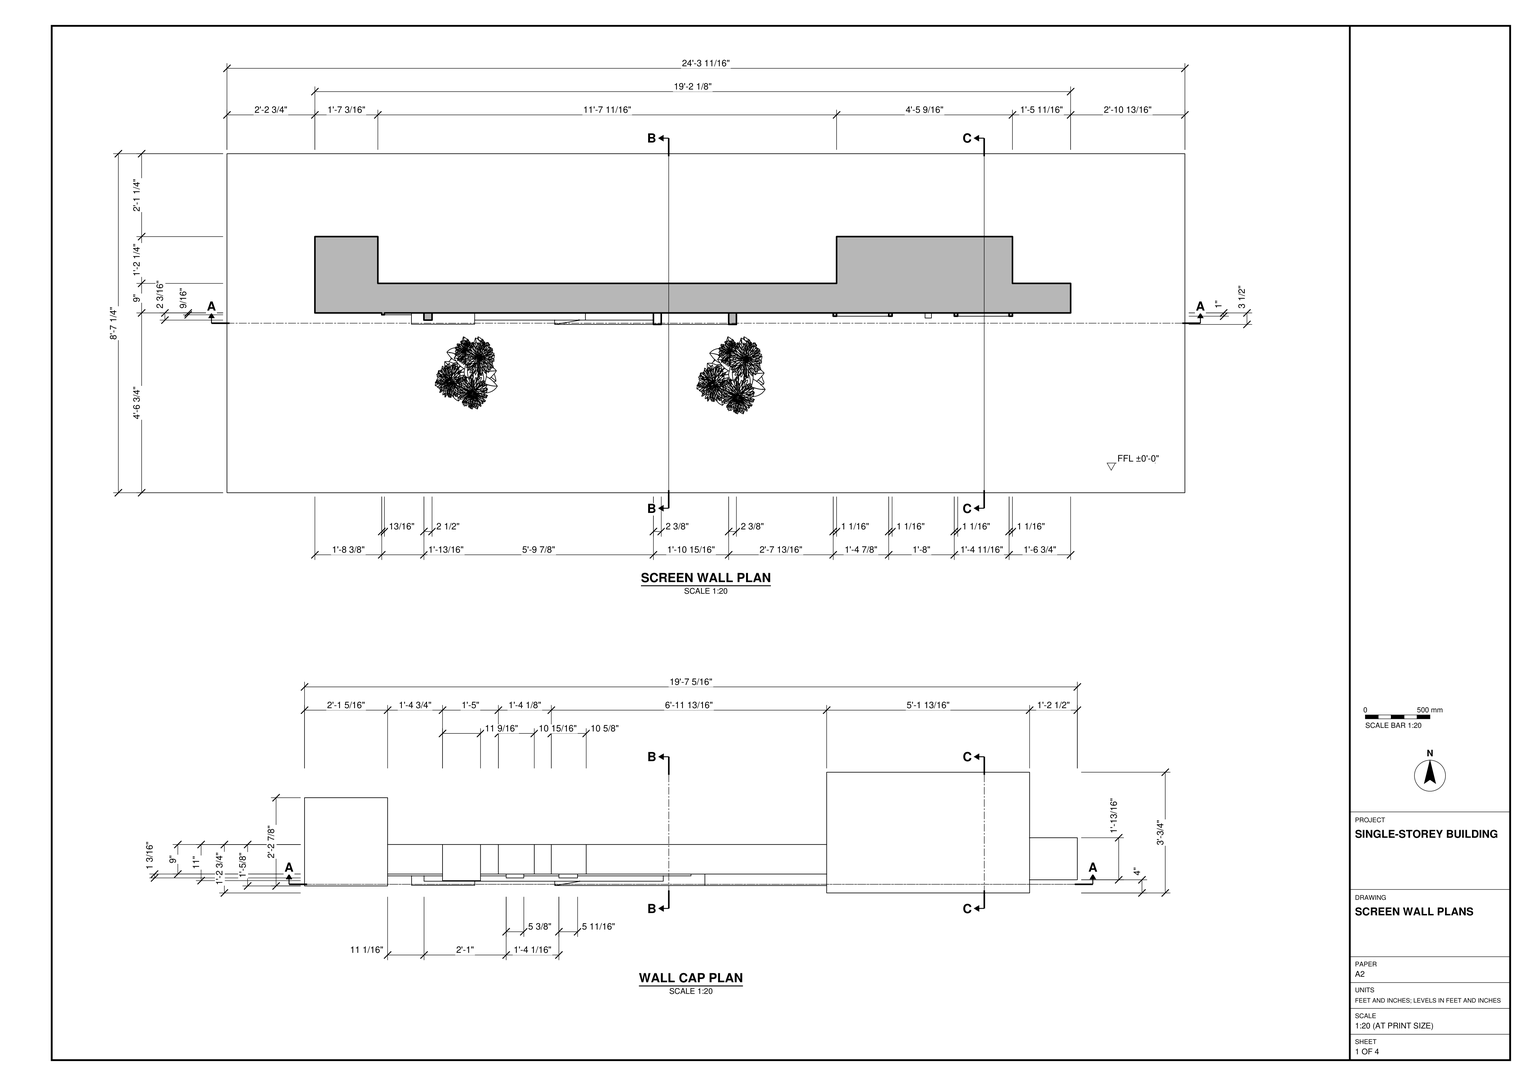
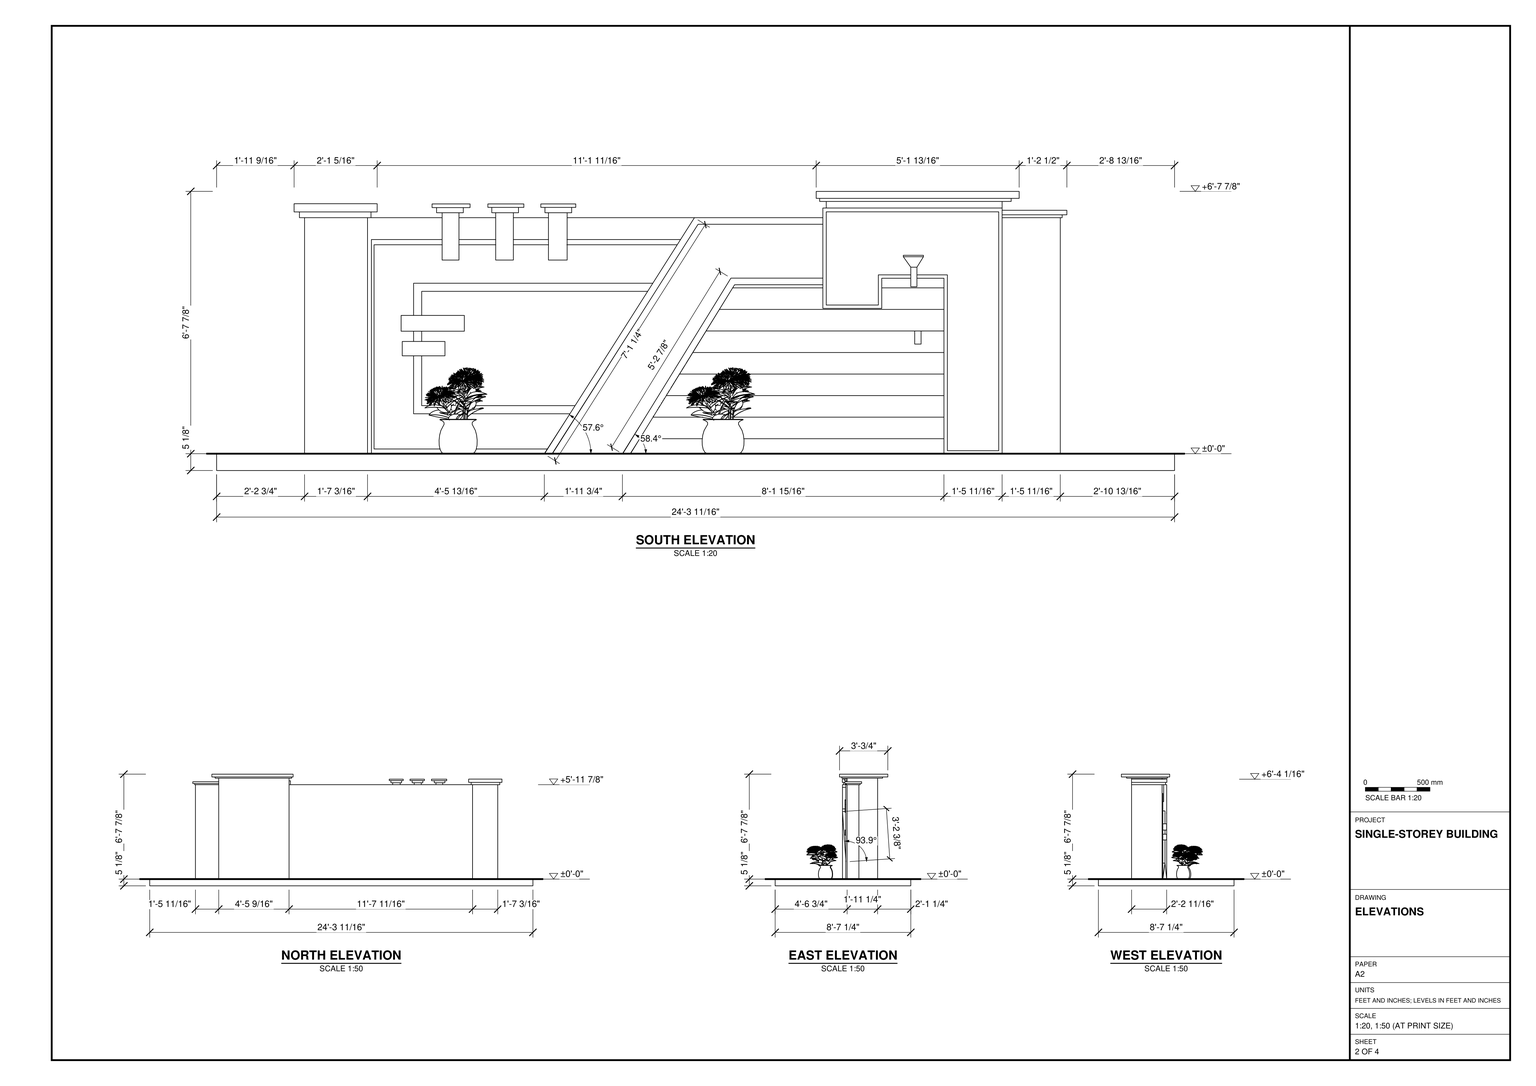
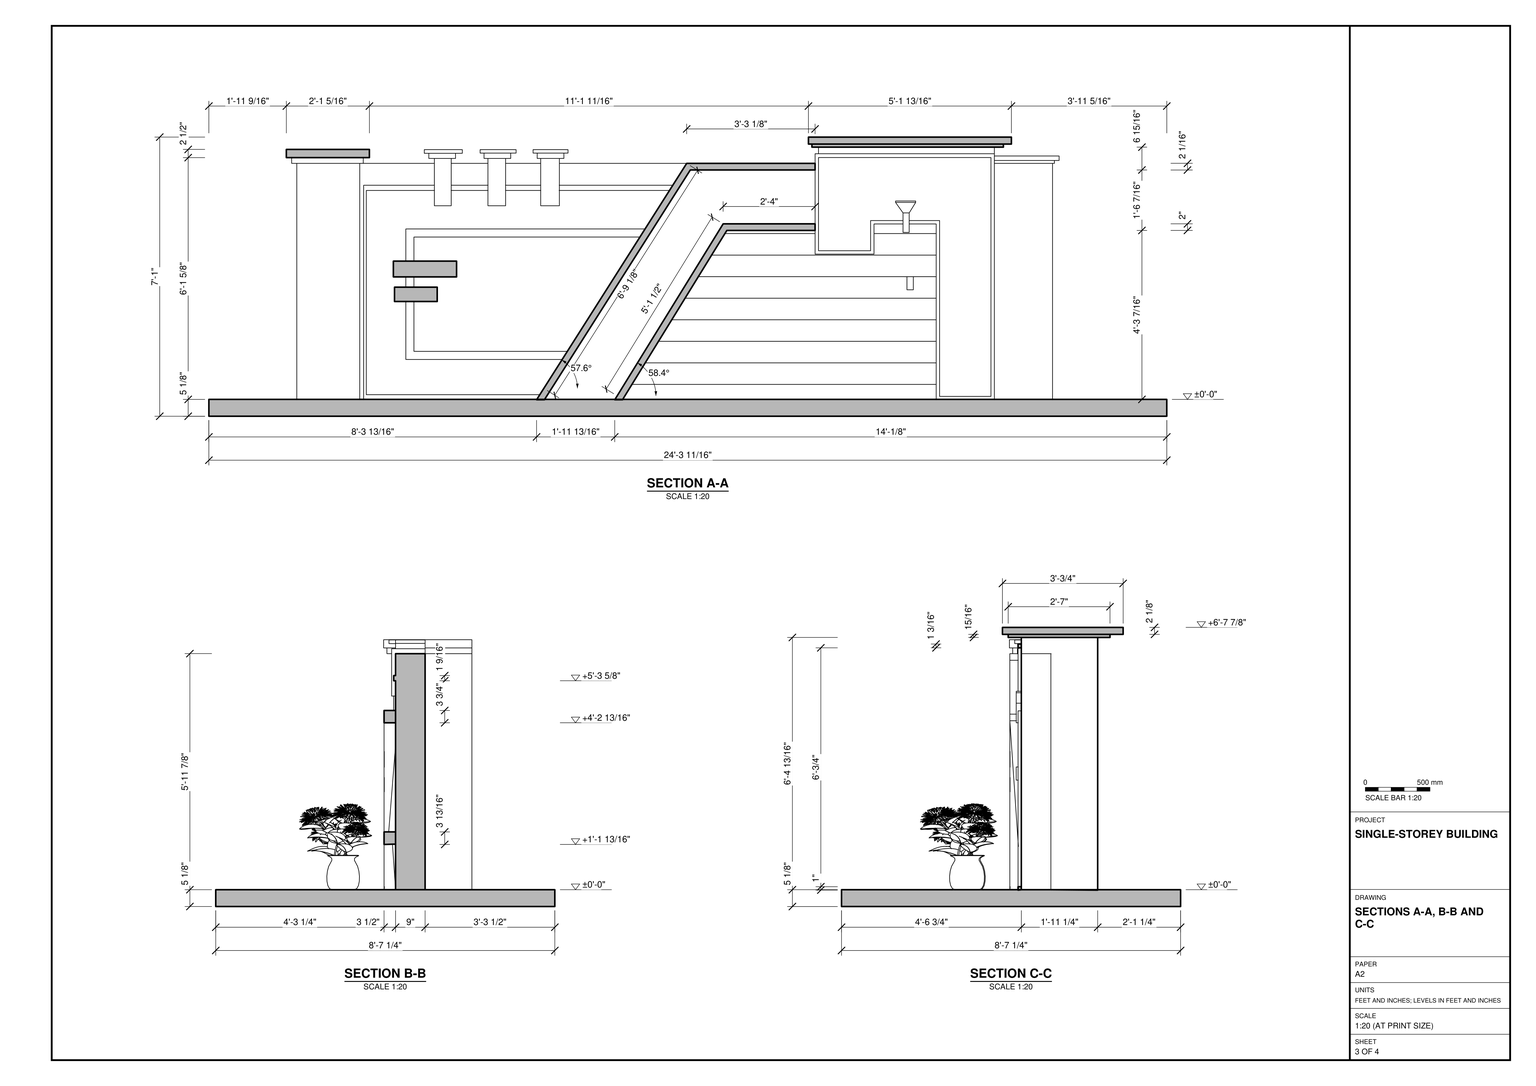
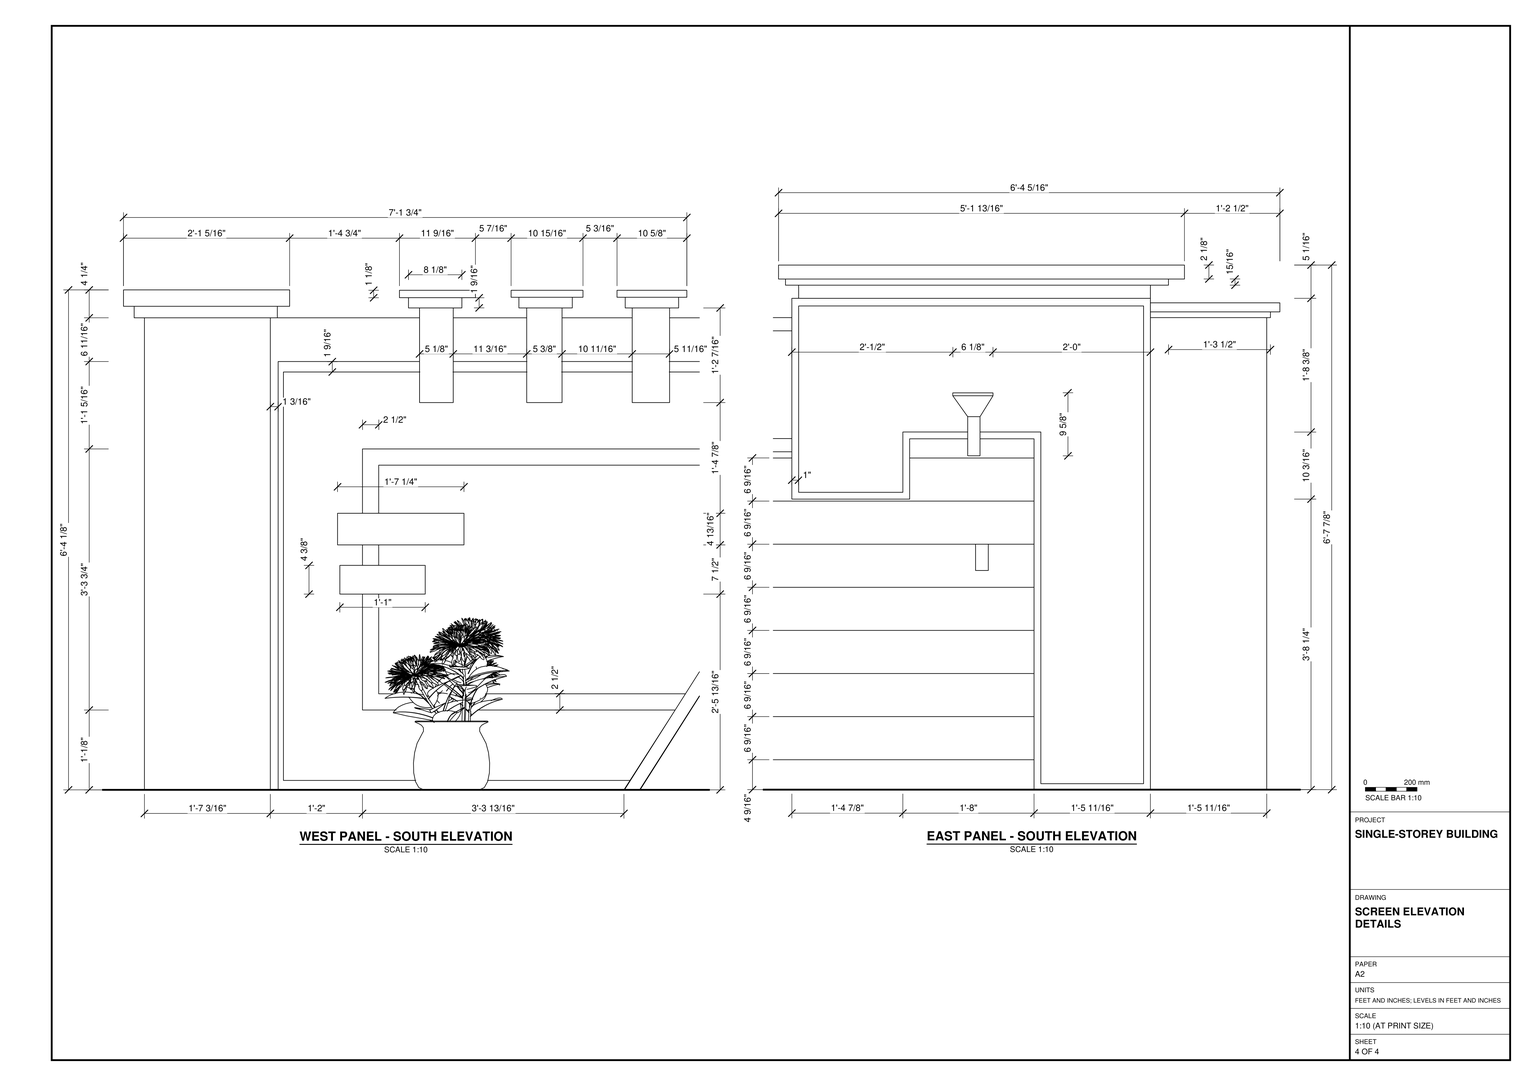
Build the screen wall and its base in SketchUp using task_files/diagram_01.pdf. Work in feet and inches. Set the top of the slab at the finished ground level of ±0'-0". The overall model is 24'-3 11/16" long, 8'-7 1/4" deep and 7'-1" high, measured from the underside of the slab to the top of the highest wall cap.

Use the screen wall plan to locate the wall on the slab and set its thicknesses. The narrow wall is deeper at the left pier and at the broad pier near the right end. Use the separate cap plan and the sections to model the cap overhangs and changes in height. On the south face, form the outlined left panel, its two short projecting bars and the three capped vertical strips above it. Run the broad diagonal band up from the slab and turn it horizontally toward the broad pier. Fit the horizontal courses beneath it to the diagonal edge and the stepped outline of the pier.

Place the two potted plants on the slab in front of the wall as shown in plan. Decor and loose items such as the plants may be any suitable library components. Keep the slab, wall and applied details in separate groups or components, and use components for repeated parts. Save one SketchUp model as output_files/freestanding_screen_wall_on_a_rectangular_slab.skp.

# SketchUp Ruby script. Lengths in inches.
U = 1.inch
M = Sketchup.active_model
def pt(a) = Geom::Point3d.new(a.map { |v| v * U })
def face(e, loops, mat)
  f = e.add_face(loops[0].map { |a| pt(a) })
  loops[1..].each { |l| e.add_face(l.map { |a| pt(a) }).erase! }
  f.material = f.back_material = mat if mat
  f
end
# faces: each face lists its corners as indices into pts; further lists are holes
def faces(e, pts, list, mat = nil) = list.each { |f| face(e, (f[0].is_a?(Array) ? f : [f]).map { |l| l.map { |i| pts[i] } }, mat) }
# xy, xz, yz: faces in a plane at the given z, y or x. An outline is a flat list of corners, or four numbers for a rectangle; further outlines are holes
def ring(l) = l.size == 4 ? [[l[0], l[1]], [l[2], l[1]], [l[2], l[3]], [l[0], l[3]]] : l.each_slice(2).to_a
def flat(e, list, mat, &to3) = list.each { |f| face(e, (f[0].is_a?(Array) ? f : [f]).map { |l| ring(l).map { |u, v| to3.(u, v) } }, mat) }
def xy(e, z, list, mat = nil) = flat(e, list, mat) { |x, y| [x, y, z] }
def xz(e, y, list, mat = nil) = flat(e, list, mat) { |x, z| [x, y, z] }
def yz(e, x, list, mat = nil) = flat(e, list, mat) { |y, z| [x, y, z] }
def lines(e, pts, list) = list.each { |a, b| e.add_line(pt(pts[a]), pt(pts[b])) }
# prism: a flat outline (further loops are holes) pulled along v
def prism(e, loops, v, mat = nil)
  f = face(e, loops, mat); d = Geom::Vector3d.new(v.map { |x| x * U })
  f.pushpull(f.normal.samedirection?(d) ? d.length : -d.length)
end
def box(e, o, s, mat = nil) = prism(e, [[o, [o[0] + s[0], o[1], o[2]], [o[0] + s[0], o[1] + s[1], o[2]], [o[0], o[1] + s[1], o[2]]]], [0, 0, s[2]], mat)
def at(x, y, z, deg = 0) = Geom::Transformation.translation(pt([x, y, z])) * Geom::Transformation.rotation(ORIGIN, Z_AXIS, deg.degrees)
def axes(o, x, y, z) = Geom::Transformation.new([*x, 0, *y, 0, *z, 0, *pt(o).to_a, 1])
def part(name) = M.definitions.add(name)
# library, detail: a bought-in or finely detailed component or shape, given as its bounding box
def library(name, o, s) = part(name).tap { |d| box(d.entities, o, s) }
def detail(e, o, s) = box(e.add_group.entities, o, s)
def put(e, d, t, mat = nil) = e.add_instance(d, t).tap { |i| i.material = mat if mat }
def group(e, t, mat = nil) = e.add_group.tap { |g| g.transformation = t; g.material = mat if mat }.entities
root = M.entities
M.materials.add("[Carrera Marble]").color = [207, 207, 207]
M.materials.add("[Color C08]").color = [102, 51, 0]
M.materials.add("[Concrete Aggregate Smoke]").color = [154, 150, 148]
c1 = library("VASO COM FLORES",[0.59,-0.39,0],[11.65,11.91,19.45])
xy(root,3.0625,[[0,0,291.6875,103.25]],"[Concrete Aggregate Smoke]")
xy(root,8.1875,[[99.78,54.1875,102.16,54.75,99.78,54.75]])
xy(root,8.1875,[[[0,0,291.6875,103.25],[47.13,54.1875,47.13,54.75,26.77,54.75,26.77,78,45.94,78,45.94,63.75,256.9,63.75,256.9,54.75,102.16,54.75,99.78,54.1875]],[47.13,54.1875,99.78,54.1875,99.78,54.75,256.9,54.75,256.9,63.75,45.94,63.75,45.94,78,26.77,78,26.77,54.75,47.13,54.75]],"[Concrete Aggregate Smoke]")
xy(root,9.1,[[222.51,53.75,238.15,54.75]])
xy(root,9.62,[[47.9375,54.1875,100.77,54.75]])
xy(root,20.34,[[59.97,52.5625,107.58,54.75]])
xy(root,22.8125,[[62.44,52.5625,109.14,54.75]])
xy(root,37.99,[[56.53,51.3125,56.53,54.75,59.97,54.75,59.97,52.5625,62.44,52.5625,62.44,54.75,69.53,54.75,69.53,51.3125]])
xy(root,41.5625,[[212.57,53.1875,214.51,54.75]],"[Carrera Marble]")
xy(root,42.37,[[56.53,51.3125,69.53,51.3125,69.53,54.75,62.44,54.75,62.44,52.5625,59.97,52.5625,59.97,54.75,56.53,54.75]])
xy(root,45.48,[[56.18,51.3125,56.18,54.75,59.97,54.75,59.97,52.5625,62.44,52.5625,62.44,54.75,75.43,54.75,75.43,51.3125]])
xy(root,45.5625,[[212.57,53.1875,214.51,54.75]],"[Carrera Marble]")
xy(root,50.3,[[56.18,51.3125,75.43,51.3125,75.43,54.75,62.44,54.75,62.44,52.5625,59.97,52.5625,59.97,54.75,56.18,54.75]])
xy(root,52.43,[[184.6,53.75,202.53,54.75]])
xy(root,53.46,[[185.63,53.75,201.5,54.75]])
xy(root,57.625,[[62.44,52.5625,131.24,54.75]])
xy(root,59.02,[[211.37,53.1875,213.25,54.75]],"[Carrera Marble]")
xy(root,59.64,[[157.72,51.25,184.6,54.75]])
xy(root,60.09,[[59.97,52.5625,132.8125,54.75]])
xy(root,61.61,[[202.53,53.75,211.37,54.75],[211.37,53.75,213.25,54.75],[213.25,53.75,221.47,54.75]])
xy(root,61.65,[[156.6,51.25,184.6,54.75]])
xy(root,62.65,[[201.5,53.75,211.37,54.75],[211.37,53.75,213.25,54.75],[213.25,53.75,222.51,54.75]])
xy(root,64.98,[[211.37,53.1875,213.25,54.75]])
xy(root,67.15,[[68.66,53.5625,73.79,54.625],[84.98,53.5625,90.36,54.75],[101.04,53.5625,106.73,54.75]])
xy(root,68.17,[[209.1,53.1875,215.22,54.75]])
xy(root,68.61,[[209.1,53.1875,215.22,54.75]],"[Carrera Marble]")
xy(root,71.8125,[[47.9375,54.1875,47.9375,54.75,140.25,54.75,140.25,54.1875,73.79,54.1875,73.79,54.625,68.66,54.625,68.66,54.1875],[68.66,54.1875,73.79,54.625]])
xy(root,73.4,[[47.13,54.1875,68.66,54.75],[68.66,54.1875,73.79,54.75],[73.79,54.1875,141.26,54.75]])
xy(root,78.05,[[146.6,51.25,184.6,54.75]])
xy(root,80.0625,[[145.49,51.25,184.6,54.75],[25.21,54.75,26.77,78],[26.77,54.75,26.77,78,45.94,78,45.94,63.75,47.01,63.75,47.01,54.75],[47.01,54.75,68.66,63.75],[68.66,54.75,73.79,63.75],
  [73.79,54.75,84.98,63.75],[84.98,54.75,90.36,63.75],[90.36,54.75,101.04,63.75],[101.04,54.75,106.73,63.75],[106.73,54.75,185.63,63.75],
  [45.94,63.75,47.01,78]])
xy(root,80.0625,[[25.21,52.125,45.94,54.75],[45.94,52.125,47.01,54.75],[239.18,54.1875,257.46,54.75],[239.18,54.75,256.9,63.75],[256.9,54.75,257.46,64.6875],
  [239.18,63.75,256.9,64.6875]],"[Carrera Marble]")
xy(root,80.9375,[[239.18,53,239.18,54.1875,257.46,54.1875,257.46,64.6875,239.18,64.6875,239.18,65.8125,258.9,65.8125,258.9,53],[239.18,54.1875,257.46,64.6875]],"[Carrera Marble]")
xy(root,81.5625,[[68.66,53.5625,73.79,54.75],[84.98,53.5625,90.36,54.75],[101.04,53.5625,106.73,54.75],[68.66,54.75,73.79,63.75],[84.98,54.75,90.36,63.75],
  [101.04,54.75,106.73,63.75]])
xy(root,81.5625,[[66.98,54.75,68.66,63.75],[73.79,54.75,75.11,63.75],[83.79,54.75,84.98,63.75],[90.36,54.75,91.92,63.75],[99.98,54.75,101.04,63.75],
  [106.73,54.75,108.11,63.75]],"[Carrera Marble]")
xy(root,81.8125,[[25.21,52.125,47.01,78]])
xy(root,81.8125,[[23.59,51.125,23.59,78,25.21,78,25.21,52.125,26.77,52.125,26.77,51.125],[26.77,51.125,45.94,52.125],[45.94,51.125,45.94,52.125,47.01,52.125,47.01,78,48.88,78,48.88,51.125]],"[Carrera Marble]")
xy(root,81.84,[[185.63,53.75,238.15,54.75]])
xy(root,82.3125,[[239.18,53,258.9,65.8125]],"[Carrera Marble]")
xy(root,83,[[184.6,53.75,239.18,54.75]])
xy(root,83.125,[[66.98,54.75,75.11,63.75]])
xy(root,83.125,[[65.6,52.75,77.17,54.75],[65.6,54.75,66.98,63.75],[75.11,54.75,77.17,63.75]],"[Carrera Marble]")
xy(root,83.1875,[[83.79,54.75,91.92,63.75],[99.98,54.75,108.11,63.75]])
xy(root,83.1875,[[82.6,54.75,83.79,63.75],[91.92,54.75,93.54,63.75],[98.73,54.75,99.98,63.75],[108.11,54.75,109.36,63.75]],"[Carrera Marble]")
xy(root,84.25,[[65.6,52.75,77.17,63.75],[82.6,54.75,93.54,63.75],[98.73,54.75,109.36,63.75]],"[Carrera Marble]")
xy(root,84.3125,[[23.59,51.125,48.88,78]],"[Carrera Marble]")
xy(root,85,[[185.63,54.75,239.18,78]])
xy(root,85,[[[183.63,50.75,241.93,81.75],[185.63,54.75,239.18,78]]],"[Carrera Marble]")
xy(root,85.9375,[[183.63,50.75,241.93,81.75]])
xy(root,85.9375,[[[182.57,49,244.37,85.75],[183.63,50.75,241.93,81.75]]],"[Carrera Marble]")
xy(root,88.0625,[[182.57,49,244.37,85.75]],"[Carrera Marble]")
xz(root,0,[[0,3.0625,291.6875,8.1875]],"[Concrete Aggregate Smoke]")
xz(root,49,[[182.57,85.9375,244.37,88.0625]],"[Carrera Marble]")
xz(root,50.75,[[183.63,85,241.93,85.9375]],"[Carrera Marble]")
xz(root,51.125,[[23.59,81.8125,48.88,84.3125]],"[Carrera Marble]")
xz(root,51.25,[[99.78,8.0625,102.16,8.0625,146.6,78.05,184.6,78.05,184.6,80.0625,145.49,80.0625],[123.58,8.0625,125.95,8.0625,157.72,59.64,184.6,59.64,184.6,61.65,156.6,61.65]])
xz(root,51.3125,[[56.53,37.99,69.53,42.37],[56.18,45.48,75.43,50.3]])
xz(root,52.125,[[25.21,80.0625,47.01,81.8125]],"[Carrera Marble]")
xz(root,52.5625,[[59.97,20.34,107.58,20.34,109.14,22.8125,62.44,22.8125,62.44,37.99,59.97,37.99],[59.97,37.99,62.44,42.37],[59.97,42.37,62.44,45.48],[59.97,45.48,62.44,50.3],[59.97,50.3,62.44,50.3,62.44,57.625,131.24,57.625,131.92,58.6875,132.8125,60.09,59.97,60.09]])
xz(root,52.75,[[65.6,83.125,77.17,84.25]],"[Carrera Marble]")
xz(root,53,[[239.18,80.9375,258.9,82.3125]],"[Carrera Marble]")
xz(root,53.1875,[[212.57,41.5625,214.51,45.5625],[211.37,59.02,213.25,64.98],[211.37,64.98,213.25,64.98,215.22,68.17,209.1,68.17],[209.1,68.17,215.22,68.61]],"[Carrera Marble]")
xz(root,53.5625,[[68.66,67.15,73.79,81.5625],[84.98,67.15,90.36,81.5625],[101.04,67.15,106.73,81.5625]],"[Carrera Marble]")
xz(root,53.75,[[221.47,8.0625,239.18,8.0625,239.18,83,184.6,83,184.6,52.43,202.53,52.43,202.53,61.61,211.37,61.61,211.37,62.65,201.5,62.65,201.5,53.46,185.63,53.46,185.63,81.84,238.15,81.84,238.15,9.1,222.51,9.1,222.51,62.65,213.25,62.65,213.25,61.61,221.47,61.61],[211.37,61.61,213.25,62.65]])
xz(root,54.1875,[[47.13,8.1875,99.78,8.1875,100.77,9.62,47.9375,9.62,47.9375,71.8125,68.66,71.8125,68.66,73.4,47.13,73.4],[68.66,71.8125,73.79,73.4],[73.79,71.8125,140.25,71.8125,141.26,73.4,73.79,73.4]])
xz(root,54.1875,[[239.18,80.0625,257.46,80.9375]],"[Carrera Marble]")
xz(root,54.625,[[68.66,67.15,73.79,71.8125]])
xz(root,54.75,[[45.94,8.1875,47.13,8.1875,47.13,73.4,68.66,73.4,68.66,80.0625,45.94,80.0625],[99.78,8.1875,100.77,9.62,107.58,20.34,109.14,22.8125,131.24,57.625,131.92,58.6875,134.3,58.6875,130.13,52.125,102.16,8.1875],[123.58,8.1875,130.51,19.3125,132.82,19.3125,125.95,8.1875],[125.95,8.1875,132.82,19.3125,132.875,19.3125,128.83,12.75],[125.95,8.1875,221.47,8.1875,221.47,12.75,128.83,12.75],
  [221.47,8.1875,221.47,61.61,202.53,61.61,202.53,58.6875,201.5,58.6875,201.5,62.65,222.51,62.65,222.51,9.1,238.15,9.1,238.15,81.84,186.61,81.84,186.61,83,239.18,83,239.18,8.1875],[128.83,12.75,221.47,12.75,221.47,19.3125,132.875,19.3125],[130.51,19.3125,134.56,25.875,136.87,25.875,132.82,19.3125],[132.82,19.3125,136.87,25.875,136.92,25.875,132.875,19.3125],[132.875,19.3125,221.47,19.3125,221.47,25.875,136.92,25.875],
  [59.97,20.34,59.97,37.99,62.44,37.99,62.44,22.8125,109.14,22.8125,107.58,20.34],[134.56,25.875,138.6,32.4375,140.92,32.4375,136.87,25.875],[136.87,25.875,140.92,32.4375,140.96,32.4375,136.92,25.875],[136.92,25.875,221.47,25.875,221.47,32.4375,140.96,32.4375],[138.6,32.4375,142.64,39,144.97,39,140.92,32.4375],
  [140.92,32.4375,144.97,39,145.01,39,140.96,32.4375],[140.96,32.4375,221.47,32.4375,221.47,39,145.01,39],[56.53,37.99,59.97,42.37],[59.97,37.99,62.44,42.37],[62.44,37.99,69.53,42.37],
  [142.64,39,146.6875,45.5625,149.03,45.5625,144.97,39],[144.97,39,149.03,45.5625,149.05,45.5625,145.01,39],[145.01,39,221.47,39,221.47,45.5625,214.51,45.5625,214.51,41.5625,212.57,41.5625,212.57,45.5625,149.05,45.5625],[212.57,41.5625,214.51,45.5625],[59.97,42.37,62.44,46.3],
  [56.18,45.48,59.97,50.3],[62.44,45.48,75.43,50.3],[146.6875,45.5625,150.73,52.125,153.08,52.125,149.03,45.5625],[149.03,45.5625,153.08,52.125,153.09,52.125,149.05,45.5625],[149.05,45.5625,221.47,45.5625,221.47,52.125,153.09,52.125],
  [59.97,46.3,62.44,50.3],[59.97,50.3,59.97,60.09,132.8125,60.09,131.92,58.6875,131.24,57.625,62.44,57.625,62.44,50.3],[150.73,52.125,154.77,58.6875,157.13,58.6875,153.08,52.125],[153.08,52.125,157.13,58.6875,157.14,58.6875,153.09,52.125],[153.08,52.125,157.13,58.6875,157.72,59.64,157.14,58.6875,153.09,52.125],
  [153.09,52.125,221.47,52.125,221.47,58.6875,202.53,58.6875,202.53,52.43,184.6,52.43,184.6,58.6875,157.14,58.6875],[184.6,52.43,184.6,58.6875,185.63,58.6875,185.63,53.46,201.5,53.46,201.5,58.6875,202.53,58.6875,202.53,52.43],[131.92,58.6875,132.8125,60.09,136.08,65.25,138.47,65.25,134.3,58.6875],[154.77,58.6875,156.6,61.65,184.6,61.65,184.6,59.64,157.72,59.64,157.13,58.6875],[157.13,58.6875,157.72,59.64,157.14,58.6875],
  [157.14,58.6875,184.6,58.6875,184.6,59.64,157.72,59.64],[184.6,58.6875,185.63,59.64],[202.53,58.6875,221.47,58.6875,221.47,61.61,213.25,61.61,213.25,59.02,211.37,59.02,211.37,61.61,202.53,61.61],[184.6,59.64,185.63,65.25],[211.37,62.65,213.25,64.98],
  [211.37,64.98,209.1,68.17,215.22,68.17,213.25,64.98],[136.08,65.25,140.25,71.8125,142.63,71.8125,138.47,65.25],[184.6,65.25,185.63,71.8125],[84.98,67.15,90.36,71.8125],[101.04,67.15,106.73,71.8125],
  [209.1,68.17,215.22,68.61],[84.98,71.8125,90.36,73.4],[101.04,71.8125,106.73,73.4],[140.25,71.8125,141.26,73.4,145.49,80.0625,184.6,80.0625,184.6,78.05,146.6,78.05,142.63,71.8125],[184.6,71.8125,185.63,80.0625],
  [68.66,73.4,73.79,80.0625],[73.79,73.4,84.98,80.0625],[84.98,73.4,90.36,80.0625],[90.36,73.4,101.04,80.0625],[101.04,73.4,106.73,80.0625],
  [106.73,73.4,141.26,73.4,145.49,80.0625,106.73,80.0625],[184.6,80.0625,185.63,83],[185.63,81.84,186.61,83]])
xz(root,54.75,[[26.77,8.1875,45.94,80.0625],[239.18,8.1875,256.9,80.0625],[62.44,22.8125,109.14,22.8125,131.24,57.625,62.44,57.625,62.44,50.3,75.43,50.3,75.43,45.48,62.44,45.48,62.44,42.37,69.53,42.37,69.53,37.99,62.44,37.99],[66.98,81.5625,75.11,83.125],[83.79,81.5625,91.92,83.1875],
  [99.98,81.5625,108.11,83.1875],[185.63,83,239.18,85],[82.6,83.1875,93.54,84.25],[98.73,83.1875,109.36,84.25]],"[Carrera Marble]")
xz(root,54.75,[[102.16,8.1875,123.58,8.1875,130.51,19.3125,134.56,25.875,142.64,39,146.6875,45.5625,150.73,52.125,154.77,58.6875,156.6,61.65,184.6,61.65,184.6,78.05,146.6,78.05,142.63,71.8125,138.47,65.25,130.13,52.125],[222.51,9.1,238.15,9.1,238.15,81.84,185.63,81.84,185.63,53.46,201.5,53.46,201.5,62.65,211.37,62.65,211.37,64.98,209.1,68.17,209.1,68.61,215.22,68.61,215.22,68.17,213.25,64.98,213.25,62.65,222.51,62.65],[47.9375,9.62,100.77,9.62,107.58,20.34,59.97,20.34,59.97,37.99,56.53,37.99,56.53,42.37,59.97,42.37,59.97,45.48,56.18,45.48,56.18,50.3,59.97,50.3,59.97,60.09,132.8125,60.09,136.08,65.25,140.25,71.8125,106.73,71.8125,106.73,67.15,101.04,67.15,101.04,71.8125,90.36,71.8125,90.36,67.15,84.98,67.15,84.98,71.8125,47.9375,71.8125]],"[Color C08]")
xz(root,63.75,[[45.94,8.1875,185.63,80.0625]])
xz(root,63.75,[[239.18,8.1875,256.9,80.0625],[68.66,80.0625,73.79,81.5625],[84.98,80.0625,90.36,81.5625],[101.04,80.0625,106.73,81.5625],[66.98,81.5625,75.11,83.125],
  [83.79,81.5625,91.92,83.1875],[99.98,81.5625,108.11,83.1875],[65.6,83.125,77.17,84.25],[82.6,83.1875,93.54,84.25],[98.73,83.1875,109.36,84.25]],"[Carrera Marble]")
xz(root,64.6875,[[239.18,80.0625,257.46,80.9375]],"[Carrera Marble]")
xz(root,65.8125,[[239.18,80.9375,258.9,82.3125]],"[Carrera Marble]")
xz(root,78,[[185.63,8.0625,239.18,85],[26.77,8.1875,45.94,80.0625],[25.21,80.0625,47.01,81.8125],[23.59,81.8125,48.88,84.3125]],"[Carrera Marble]")
xz(root,81.75,[[183.63,85,241.93,85.9375]],"[Carrera Marble]")
xz(root,85.75,[[182.57,85.9375,244.37,88.0625]],"[Carrera Marble]")
xz(root,103.25,[[0,3.0625,291.6875,8.1875]],"[Concrete Aggregate Smoke]")
yz(root,0,[[0,3.0625,103.25,8.1875]],"[Concrete Aggregate Smoke]")
yz(root,23.59,[[51.125,81.8125,78,84.3125]],"[Carrera Marble]")
yz(root,25.21,[[52.125,80.0625,78,81.8125]],"[Carrera Marble]")
yz(root,26.77,[[54.75,8.1875,78,80.0625]],"[Carrera Marble]")
yz(root,45.94,[[63.75,8.1875,78,80.0625]],"[Carrera Marble]")
yz(root,47.01,[[52.125,80.0625,78,81.8125]],"[Carrera Marble]")
yz(root,47.13,[[54.1875,8.1875,54.75,73.4]])
yz(root,47.9375,[[54.1875,9.62,54.75,71.8125]])
yz(root,48.88,[[51.125,81.8125,78,84.3125]],"[Carrera Marble]")
yz(root,56.18,[[51.3125,45.48,54.75,50.3]])
yz(root,56.53,[[51.3125,37.99,54.75,42.37]])
yz(root,59.97,[[52.5625,20.34,54.75,37.99],[52.5625,37.99,54.75,42.37],[52.5625,42.37,54.75,45.48],[52.5625,45.48,54.75,50.3],[52.5625,50.3,54.75,60.09]])
yz(root,62.44,[[52.5625,22.8125,54.75,37.99],[52.5625,37.99,54.75,42.37],[52.5625,42.37,54.75,45.48],[52.5625,45.48,54.75,50.3],[52.5625,50.3,54.75,57.625]])
yz(root,65.6,[[52.75,83.125,63.75,84.25]],"[Carrera Marble]")
yz(root,66.98,[[54.75,81.5625,63.75,83.125]],"[Carrera Marble]")
yz(root,68.66,[[53.5625,67.15,53.5625,81.5625,63.75,81.5625,63.75,80.0625,54.75,80.0625,54.75,73.4,54.1875,73.4,54.1875,71.8125,54.625,71.8125,54.625,67.15]],"[Carrera Marble]")
yz(root,69.53,[[51.3125,37.99,54.75,42.37]])
yz(root,73.79,[[53.5625,67.15,54.625,67.15,54.625,71.8125,54.1875,71.8125,54.1875,73.4,54.75,73.4,54.75,80.0625,63.75,80.0625,63.75,81.5625,53.5625,81.5625]],"[Carrera Marble]")
yz(root,75.11,[[54.75,81.5625,63.75,83.125]])
yz(root,75.43,[[51.3125,45.48,54.75,50.3]])
yz(root,77.17,[[52.75,83.125,63.75,84.25]])
yz(root,82.6,[[54.75,83.1875,63.75,84.25]],"[Carrera Marble]")
yz(root,83.79,[[54.75,81.5625,63.75,83.1875]],"[Carrera Marble]")
yz(root,84.98,[[53.5625,67.15,53.5625,81.5625,63.75,81.5625,63.75,80.0625,54.75,80.0625,54.75,67.15]],"[Carrera Marble]")
yz(root,90.36,[[53.5625,67.15,54.75,67.15,54.75,80.0625,63.75,80.0625,63.75,81.5625,53.5625,81.5625]],"[Carrera Marble]")
yz(root,91.92,[[54.75,81.5625,63.75,83.1875]],"[Carrera Marble]")
yz(root,93.54,[[54.75,83.1875,63.75,84.25]],"[Carrera Marble]")
yz(root,98.73,[[54.75,83.1875,63.75,84.25]],"[Carrera Marble]")
yz(root,99.98,[[54.75,81.5625,63.75,83.1875]],"[Carrera Marble]")
yz(root,101.04,[[53.5625,67.15,53.5625,81.5625,63.75,81.5625,63.75,80.0625,54.75,80.0625,54.75,67.15]],"[Carrera Marble]")
yz(root,106.73,[[53.5625,67.15,54.75,67.15,54.75,80.0625,63.75,80.0625,63.75,81.5625,53.5625,81.5625]],"[Carrera Marble]")
yz(root,108.11,[[54.75,81.5625,63.75,83.1875]],"[Carrera Marble]")
yz(root,109.36,[[54.75,83.1875,63.75,84.25]],"[Carrera Marble]")
yz(root,182.57,[[49,85.9375,85.75,88.0625]],"[Carrera Marble]")
yz(root,183.63,[[50.75,85,81.75,85.9375]],"[Carrera Marble]")
yz(root,184.6,[[53.75,52.43,54.75,59.64],[51.25,59.64,53.75,61.65],[53.75,59.64,54.75,61.65],[53.75,61.65,54.75,78.05],[51.25,78.05,53.75,80.0625],
  [53.75,78.05,54.75,80.0625],[53.75,80.0625,54.75,83]])
yz(root,185.63,[[53.75,53.46,54.75,81.84]])
yz(root,185.63,[[78,8.0625,63.75,8.1875,63.75,80.0625,54.75,80.0625,54.75,85,78,85]],"[Carrera Marble]")
yz(root,201.5,[[53.75,53.46,54.75,62.65]])
yz(root,202.53,[[53.75,52.43,54.75,61.61]])
yz(root,209.1,[[53.1875,68.17,54.75,68.61]],"[Carrera Marble]")
yz(root,211.37,[[53.1875,59.02,53.1875,64.98,54.75,64.98,54.75,62.65,53.75,62.65,53.75,61.61,54.75,61.61,54.75,59.02]],"[Carrera Marble]")
yz(root,212.57,[[53.1875,41.5625,54.75,45.5625]],"[Carrera Marble]")
yz(root,213.25,[[53.1875,59.02,54.75,59.02,54.75,61.61,53.75,61.61,53.75,62.65,54.75,62.65,54.75,64.98,53.1875,64.98]],"[Carrera Marble]")
yz(root,214.51,[[53.1875,41.5625,54.75,45.5625]],"[Carrera Marble]")
yz(root,215.22,[[53.1875,68.17,54.75,68.61]],"[Carrera Marble]")
yz(root,221.47,[[53.75,8.0625,53.75,61.61,54.75,61.61,54.75,8.1875]])
yz(root,222.51,[[53.75,9.1,54.75,62.65]])
yz(root,238.15,[[53.75,9.1,54.75,81.84]])
yz(root,239.18,[[53.75,8.0625,54.75,8.1875,54.75,80.0625,54.1875,80.0625,54.1875,80.9375,53.75,80.9375],[53.75,80.9375,54.75,82.3125],[53.75,82.3125,54.75,83]])
yz(root,239.18,[[78,8.0625,78,85,54.75,85,54.75,82.3125,65.8125,82.3125,65.8125,80.9375,64.6875,80.9375,64.6875,80.0625,63.75,80.0625,63.75,8.1875],[54.1875,80.0625,54.75,80.9375],[54.75,80.0625,64.6875,80.9375],[53,80.9375,53.75,82.3125],[54.75,80.9375,65.8125,82.3125]],"[Carrera Marble]")
yz(root,241.93,[[50.75,85,81.75,85.9375]],"[Carrera Marble]")
yz(root,244.37,[[49,85.9375,85.75,88.0625]],"[Carrera Marble]")
yz(root,256.9,[[54.75,8.1875,63.75,80.0625]],"[Carrera Marble]")
yz(root,257.46,[[54.1875,80.0625,64.6875,80.9375]],"[Carrera Marble]")
yz(root,258.9,[[53,80.9375,65.8125,82.3125]],"[Carrera Marble]")
yz(root,291.6875,[[0,3.0625,103.25,8.1875]],"[Concrete Aggregate Smoke]")
p = [[99.78,51.25,8.0625],[99.78,54.1875,8.1875],[102.16,54.75,8.1875],[102.16,51.25,8.0625],[132.8125,54.75,60.09],[132.8125,52.5625,60.09],
  [131.92,52.5625,58.6875],[131.24,52.5625,57.625],[109.14,52.5625,22.8125],[107.58,52.5625,20.34],[145.49,51.25,80.0625],[145.49,54.75,80.0625],
  [141.26,54.75,73.4],[141.26,54.1875,73.4],[140.25,54.1875,71.8125],[140.25,54.75,71.8125],[136.08,54.75,65.25],[130.13,54.75,52.125],
  [134.3,54.75,58.6875],[138.47,54.75,65.25],[142.63,54.75,71.8125],[146.6,54.75,78.05],[146.6,51.25,78.05],[123.58,54.75,8.1875],
  [125.95,54.75,8.1875],[125.95,51.25,8.0625],[123.58,51.25,8.0625],[156.6,51.25,61.65],[156.6,54.75,61.65],[154.77,54.75,58.6875],
  [150.73,54.75,52.125],[146.6875,54.75,45.5625],[142.64,54.75,39],[138.6,54.75,32.4375],[134.56,54.75,25.875],[130.51,54.75,19.3125],
  [157.72,51.25,59.64],[221.47,54.75,8.1875],[239.18,54.75,8.1875],[239.18,53.75,8.0625],[221.47,53.75,8.0625],[185.63,78,8.0625],
  [239.18,78,8.0625],[239.18,63.75,8.1875],[185.63,63.75,8.1875],[157.72,54.75,59.64],[132.82,54.75,19.3125],[136.87,54.75,25.875],
  [140.92,54.75,32.4375],[144.97,54.75,39],[149.03,54.75,45.5625],[153.08,54.75,52.125],[157.13,54.75,58.6875],[100.77,54.1875,9.62],
  [100.77,54.75,9.62],[99.78,54.75,8.1875],[107.58,54.75,20.34],[109.14,54.75,22.8125],[131.24,54.75,57.625],[131.92,54.75,58.6875],
  [209.1,54.75,68.17],[211.37,54.75,64.98],[211.37,53.1875,64.98],[209.1,53.1875,68.17],[213.25,54.75,64.98],[215.22,54.75,68.17],
  [215.22,53.1875,68.17],[213.25,53.1875,64.98],[128.83,54.75,52.125]]
faces(root,p,[[0,1,2],[3,0,2],[4,5,6,7,8,9,0,10,11,12,13,14,15,16],[1,0,9],[3,2,17],[18,19,20,21,22,3,17],[23,24,25,26],[27,28,29,30,31,32,33,34,35,26],
  [23,26,35],[25,24,36],[37,38,39,40],[41,42,43,44],[45,36,24,46,47,48,49,50,51,52],[53,1,9],[53,54,55,1],[9,56,54,53],
  [57,56,9,8],[57,8,7,58],[59,58,7,6],[4,59,6,5],[12,15,14,13]])
faces(root,p,[[60,61,62,63],[64,65,66,67]],"[Carrera Marble]")
lines(root,p,[[68,17]])
put(root,c1,axes([62.4375,26.21,8.1875],[1.6256,0,0],[0,1.8492,0],[0,0,1.35]))
put(root,c1,axes([142.01,24.77,8.1875],[1.78816,0,0],[0,1.9734,0],[0,0,1.35]))
